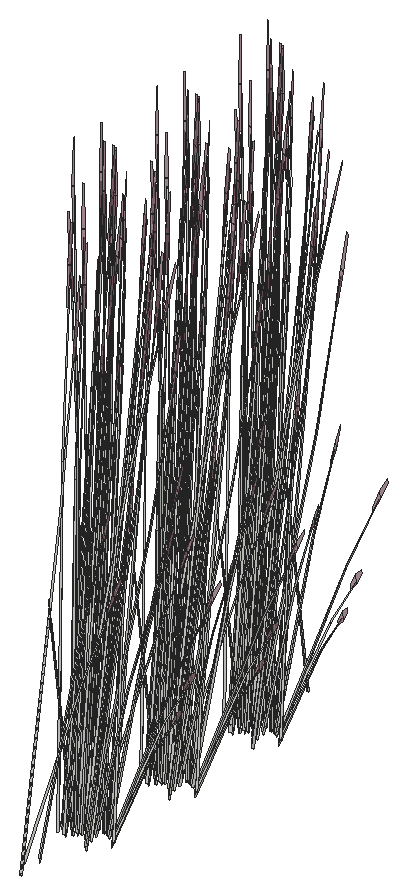
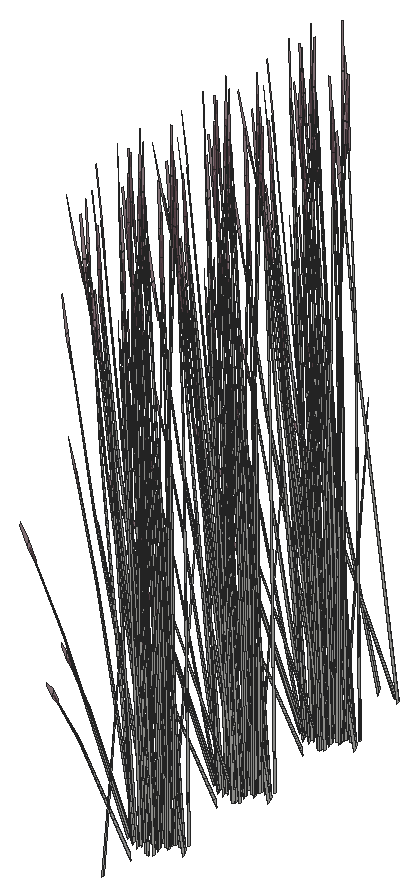
# SketchUp Ruby script. Lengths in inches.
U = 1.inch
M = Sketchup.active_model
def pt(a) = Geom::Point3d.new(a.map { |v| v * U })
def face(e, loops, mat)
  f = e.add_face(loops[0].map { |a| pt(a) })
  loops[1..].each { |l| e.add_face(l.map { |a| pt(a) }).erase! }
  f.material = f.back_material = mat if mat
  f
end
# faces: each face lists its corners as indices into pts; further lists are holes
def faces(e, pts, list, mat = nil) = list.each { |f| face(e, (f[0].is_a?(Array) ? f : [f]).map { |l| l.map { |i| pts[i] } }, mat) }
# xy, xz, yz: faces in a plane at the given z, y or x. An outline is a flat list of corners, or four numbers for a rectangle; further outlines are holes
def ring(l) = l.size == 4 ? [[l[0], l[1]], [l[2], l[1]], [l[2], l[3]], [l[0], l[3]]] : l.each_slice(2).to_a
def flat(e, list, mat, &to3) = list.each { |f| face(e, (f[0].is_a?(Array) ? f : [f]).map { |l| ring(l).map { |u, v| to3.(u, v) } }, mat) }
def xy(e, z, list, mat = nil) = flat(e, list, mat) { |x, y| [x, y, z] }
def xz(e, y, list, mat = nil) = flat(e, list, mat) { |x, z| [x, y, z] }
def yz(e, x, list, mat = nil) = flat(e, list, mat) { |y, z| [x, y, z] }
def lines(e, pts, list) = list.each { |a, b| e.add_line(pt(pts[a]), pt(pts[b])) }
# prism: a flat outline (further loops are holes) pulled along v
def prism(e, loops, v, mat = nil)
  f = face(e, loops, mat); d = Geom::Vector3d.new(v.map { |x| x * U })
  f.pushpull(f.normal.samedirection?(d) ? d.length : -d.length)
end
def box(e, o, s, mat = nil) = prism(e, [[o, [o[0] + s[0], o[1], o[2]], [o[0] + s[0], o[1] + s[1], o[2]], [o[0], o[1] + s[1], o[2]]]], [0, 0, s[2]], mat)
def at(x, y, z, deg = 0) = Geom::Transformation.translation(pt([x, y, z])) * Geom::Transformation.rotation(ORIGIN, Z_AXIS, deg.degrees)
def axes(o, x, y, z) = Geom::Transformation.new([*x, 0, *y, 0, *z, 0, *pt(o).to_a, 1])
def part(name) = M.definitions.add(name)
# library, detail: a bought-in or finely detailed component or shape, given as its bounding box
def library(name, o, s) = part(name).tap { |d| box(d.entities, o, s) }
def detail(e, o, s) = box(e.add_group.entities, o, s)
def put(e, d, t, mat = nil) = e.add_instance(d, t).tap { |i| i.material = mat if mat }
def group(e, t, mat = nil) = e.add_group.tap { |g| g.transformation = t; g.material = mat if mat }.entities
root = M.entities
M.materials.add("LightPink_Translucent").color = [144, 107, 117]
M.materials["LightPink_Translucent"].alpha = 0.75
c1 = part("blade")
p = [[2.15,0.21,22],[0,0.17,0],[0.09,0.45,0],[2.18,0.31,22],[2.29,0.31,22],[0.38,0.45,0],
  [2.48,0.24,33],[2.49,0.24,33],[2.48,0.22,33]]
faces(c1.entities,p,[[0,1,2,3],[4,5,2,3],[6,3,4,7],[8,0,3,6]])
c2 = part("seeds")
p = [[0.3,-0.1,1.38],[-0.01,-0.03,1.59],[-0.01,-0.03,0.03],[0.14,-0.07,-0.07],[0.29,-0.03,3],[0.15,0.01,3.11]]
faces(c2.entities,p,[[0,1,2,3],[1,0,4,5]],"LightPink_Translucent")
c3 = part("blade with seeds")
put(c3.entities,c1,at(0,0,0))
put(c3.entities,c2,axes([2.4,0.25,30.99],[1.5799,-0.05474,1.17369],[-0.12525,1.92788,0.29478],[-0.07173,-0.02425,1.56792]))
put(root,c3,axes([334.9,443.32,49.85],[0.18514,0.35777,-0.61156],[-0.53331,0.12885,-0.16051],[0.02046,0.12115,1.3499]))
put(root,c3,axes([335.47,444.69,50.36],[-0.32378,-0.01225,0.92831],[0.21383,-0.26028,0.51254],[0.12791,0.09247,0.72818]))
put(root,c3,axes([334.77,449.54,50.29],[-0.14352,0.07909,1.26356],[-0.42983,-0.13843,-0.27174],[0.07968,-0.17216,0.54024]))
put(root,c3,axes([334.42,444.06,50.29],[0.00891,-0.12953,1.26356],[0.4258,-0.14469,-0.27174],[0.13144,0.15503,0.54024]))
put(root,c3,axes([335.77,449.78,49.32],[-0.07557,-0.03078,1.55816],[-0.19412,-0.34391,-0.23804],[0.13095,-0.09333,0.26541]))
put(root,c3,axes([332.92,449.85,50.1],[-0.31568,-0.39156,0],[0.52815,-0.21836,-0.456],[0.12029,-0.04973,1.44655]))
put(root,c3,axes([333.35,449.79,49.78],[0.47255,-0.19538,-0.43871],[0.28245,0.35034,0],[0.10763,-0.0445,1.3917]))
put(root,c3,axes([336.15,450.47,50.29],[-0.18038,-0.01157,1.26356],[-0.18479,-0.31048,-0.27174],[0.22159,-0.08783,0.54024]))
put(root,c3,axes([333.91,450.6,49.82],[0.34009,-0.2937,-0.55095],[0.42248,0.26632,-0.1446],[0.13628,-0.07327,1.21613]))
put(root,c3,axes([333.54,450.9375,50.36],[-0.05884,-0.44587,-0.25709],[0.6128,-0.02696,-0.44182],[0.10791,-0.05939,1.41118]))
put(root,c3,axes([333.46,449.95,49.79],[0.47106,0.09668,-0.27372],[-0.11861,0.34048,0.27372],[0.09497,-0.03926,1.22797]))
put(root,c3,axes([333.62,451.29,50.15],[0.56891,0.18939,0.21263],[-0.2738,0.39352,0.44182],[0,-0.09071,1.41855]))
put(root,c3,axes([333.44,451.02,50.4],[-0.54829,0.02412,0.39531],[-0.04958,-0.40041,-0.19025],[0.09816,-0.04058,1.26923]))
put(root,c3,axes([335.24,449.95,50.1],[0.31568,-0.39156,0],[0.52815,0.21836,-0.456],[0.12029,0.04973,1.44655]))
put(root,c3,axes([336.49,451.5,49.75],[-0.3252,0.04689,1.25103],[-0.05176,-0.37326,0.07161],[0.22777,-0.0565,0.71188]))
put(root,c3,axes([337.08,451.17,50],[-0.31304,-0.24986,-0.05733],[0.34284,-0.22894,-0.25992],[0.09714,-0.01612,0.85731]))
put(root,c3,axes([334.21,451.2,49.95],[0,-0.45213,0],[0.63136,0,0],[0,0,1.58567]))
put(root,c3,axes([334.97,450.16,50.19],[-0.47255,-0.19538,0.43871],[0.28245,-0.35034,0],[0.10763,0.0445,1.3917]))
put(root,c3,axes([333.91,450.92,50.09],[-0.41865,0.35461,0.40429],[-0.49737,-0.31303,0.15865],[0.10093,-0.03539,1.40366]))
put(root,c3,axes([333.18,450.33,50.1875],[-0.14586,0.38834,0.15589],[-0.53375,-0.1099,0.31002],[0.0922,-0.00189,1.41735]))
put(root,c3,axes([332.96,450.65,49.41],[-0.49699,0.15644,1.13921],[-0.15819,-0.44887,0.44265],[0.30518,0.00747,1.29573]))
put(root,c3,axes([334.29,450.77,50.3125],[0.09741,-0.34873,0.12794],[0.4759,0.06053,-0.36534],[0.08661,0.03581,1.11991]))
put(root,c3,axes([336.84,451.26,49.32],[-0.02639,-0.05932,1.55816],[0.18302,-0.34702,-0.23804],[0.18462,-0.00499,0.26541]))
put(root,c3,axes([334.09,450.86,50.4],[-0.30332,-0.32798,0.39531],[0.45944,-0.23096,-0.19025],[0.09816,0.04058,1.26923]))
put(root,c3,axes([334.25,450.88,50.36],[0.50979,-0.25942,-0.25709],[0.339,0.36656,-0.44182],[0.12578,0.03723,1.41118]))
put(root,c3,axes([335.53,450.1875,49.78],[0.47255,0.19538,-0.43871],[-0.28245,0.35034,0],[0.10763,0.0445,1.3917]))
put(root,c3,axes([334.63,451.3,49.95],[0.56491,0,0],[0,0.40454,0],[0,0,1.5764]))
put(root,c3,axes([334.79,450.36,50.1875],[-0.54257,0.10371,0.15589],[-0.13397,-0.38597,0.31002],[0.04839,0.05624,1.41735]))
put(root,c3,axes([335.4,450.34,49.79],[0.11861,0.34048,-0.27372],[-0.47106,0.09668,0.27372],[0.09497,0.03926,1.22797]))
put(root,c3,axes([334.45,451.1,50.1],[-0.63817,-0.08233,0.43472],[0.12987,-0.46497,0.17059],[0.09326,0.0449,1.50931]))
put(root,c3,axes([334.56,452.2,49.93],[0.53009,-0.13258,-0.16963],[0.18627,0.38191,0.00007],[0.05851,-0.01465,1.53656]))
put(root,c3,axes([334.62,451.48,49.96],[0.35245,0.2524,0],[-0.35245,0.2524,0],[0,0,1.49564]))
put(root,c3,axes([335.58,451.37,50.1875],[-0.39671,-0.28463,0.15589],[0.39978,-0.27607,0.31002],[-0.04381,0.05813,1.41735]))
put(root,c3,axes([334.84,450.9375,49.82],[0.52523,0.06406,-0.55095],[-0.11084,0.39517,-0.1446],[0.15674,0.04788,1.21613]))
put(root,c3,axes([334.62,451.18,50.4],[0.24498,-0.3521,0.39531],[0.50902,0.16945,-0.19025],[0,0.08116,1.26923]))
put(root,c3,axes([334.52,451.38,50.03],[0,0.45191,-0.04981],[-0.63136,0,0],[0,0.0142,1.58489]))
put(root,c3,axes([334.57,451.0625,49.95],[0.30332,0.32798,-0.39531],[-0.45944,0.23096,0.19025],[0.09816,0.04058,1.26923]))
put(root,c3,axes([335.9,451.38,50.19],[0,-0.39075,0.43871],[0.56491,0,0],[0,0.089,1.3917]))
put(root,c3,axes([334.83,451.26,50.3125],[0.47043,-0.11396,0.12794],[0.16474,0.32541,-0.36534],[0,0.07162,1.11991]))
put(root,c3,axes([336.58,452.06,50.29],[-0.1216,-0.0961,1.26356],[0.15822,-0.31792,-0.27174],[0.24603,0.04307,0.54024]))
put(root,c3,axes([334.4,452.41,49.95],[0.50902,0.17543,0],[-0.24498,0.36452,0],[0,0,1.54589]))
put(root,c3,axes([334.22,452.26,50.02],[0.21952,0.44891,-0.05313],[-0.62724,0.1573,0],[0.00767,0.01568,1.52132]))
put(root,c3,axes([336.29,451.44,50.1],[0.63136,0,0],[0,0.43672,-0.456],[0,0.09947,1.44655]))
put(root,c3,axes([336.03,451.67,49.94],[-0.63105,-0.00312,-0.04397],[0,-0.43672,0.44129],[-0.01983,0.09942,1.3992]))
put(root,c3,axes([334.67,451.29,50.36],[0.56863,0.18645,-0.25709],[-0.2738,0.39352,-0.44182],[0.01787,0.09662,1.41118]))
put(root,c3,axes([335.9,451.73,49.79],[-0.35245,0.2438,-0.27372],[-0.35245,-0.2438,0.27372],[0,0.07853,1.22797]))
put(root,c3,axes([334.61,451.58,49.95],[-0.24498,0.3521,-0.39531],[-0.50902,-0.16945,0.19025],[0,0.08116,1.26923]))
put(root,c3,axes([336.15,451.74,49.78],[0,0.39075,-0.43871],[-0.56491,0,0],[0,0.089,1.3917]))
put(root,c3,axes([335.51,452.97,49.32],[0.03679,-0.05641,1.55816],[0.46313,-0.16615,-0.23804],[0.14041,0.08599,0.26541]))
put(root,c3,axes([334.9,451.6875,49.85],[0.18514,0.35777,-0.61156],[-0.53331,0.12885,-0.16051],[0.02046,0.12115,1.3499]))
put(root,c3,axes([335.47,453.0625,50.36],[-0.32378,-0.01225,0.92831],[0.21383,-0.26028,0.51254],[0.12791,0.09247,0.72818]))
put(root,c3,axes([334.42,452.43,50.29],[0.00891,-0.12953,1.26356],[0.4258,-0.14469,-0.27174],[0.13144,0.15503,0.54024]))
put(root,c3,axes([334.77,459.05,50.29],[-0.14352,0.07909,1.26356],[-0.42983,-0.13843,-0.27174],[0.07968,-0.17216,0.54024]))
put(root,c3,axes([335.77,459.3,49.32],[-0.07557,-0.03078,1.55816],[-0.19412,-0.34391,-0.23804],[0.13095,-0.09333,0.26541]))
put(root,c3,axes([332.92,459.37,50.1],[-0.31568,-0.39156,0],[0.52815,-0.21836,-0.456],[0.12029,-0.04973,1.44655]))
put(root,c3,axes([333.35,459.31,49.78],[0.47255,-0.19538,-0.43871],[0.28245,0.35034,0],[0.10763,-0.0445,1.3917]))
put(root,c3,axes([336.15,459.98,50.29],[-0.18038,-0.01157,1.26356],[-0.18479,-0.31048,-0.27174],[0.22159,-0.08783,0.54024]))
put(root,c3,axes([333.91,460.11,49.82],[0.34009,-0.2937,-0.55095],[0.42248,0.26632,-0.1446],[0.13628,-0.07327,1.21613]))
put(root,c3,axes([333.54,460.45,50.36],[-0.05884,-0.44587,-0.25709],[0.6128,-0.02696,-0.44182],[0.10791,-0.05939,1.41118]))
put(root,c3,axes([333.46,459.46,49.79],[0.47106,0.09668,-0.27372],[-0.11861,0.34048,0.27372],[0.09497,-0.03926,1.22797]))
put(root,c3,axes([333.62,460.8,50.15],[0.56891,0.18939,0.21263],[-0.2738,0.39352,0.44182],[0,-0.09071,1.41855]))
put(root,c3,axes([333.44,460.54,50.4],[-0.54829,0.02412,0.39531],[-0.04958,-0.40041,-0.19025],[0.09816,-0.04058,1.26923]))
put(root,c3,axes([335.24,459.47,50.1],[0.31568,-0.39156,0],[0.52815,0.21836,-0.456],[0.12029,0.04973,1.44655]))
put(root,c3,axes([336.49,461.02,49.75],[-0.3252,0.04689,1.25103],[-0.05176,-0.37326,0.07161],[0.22777,-0.0565,0.71188]))
put(root,c3,axes([337.08,460.68,50],[-0.31304,-0.24986,-0.05733],[0.34284,-0.22894,-0.25992],[0.09714,-0.01612,0.85731]))
put(root,c3,axes([334.21,460.72,49.95],[0,-0.45213,0],[0.63136,0,0],[0,0,1.58567]))
put(root,c3,axes([334.97,459.67,50.19],[-0.47255,-0.19538,0.43871],[0.28245,-0.35034,0],[0.10763,0.0445,1.3917]))
put(root,c3,axes([333.91,460.43,50.09],[-0.41865,0.35461,0.40429],[-0.49737,-0.31303,0.15865],[0.10093,-0.03539,1.40366]))
put(root,c3,axes([333.18,459.85,50.1875],[-0.14586,0.38834,0.15589],[-0.53375,-0.1099,0.31002],[0.0922,-0.00189,1.41735]))
put(root,c3,axes([332.96,460.16,49.41],[-0.49699,0.15644,1.13921],[-0.15819,-0.44887,0.44265],[0.30518,0.00747,1.29573]))
put(root,c3,axes([334.29,460.28,50.3125],[0.09741,-0.34873,0.12794],[0.4759,0.06053,-0.36534],[0.08661,0.03581,1.11991]))
put(root,c3,axes([336.84,460.77,49.32],[-0.02639,-0.05932,1.55816],[0.18302,-0.34702,-0.23804],[0.18462,-0.00499,0.26541]))
put(root,c3,axes([334.09,460.37,50.4],[-0.30332,-0.32798,0.39531],[0.45944,-0.23096,-0.19025],[0.09816,0.04058,1.26923]))
put(root,c3,axes([334.25,460.39,50.36],[0.50979,-0.25942,-0.25709],[0.339,0.36656,-0.44182],[0.12578,0.03723,1.41118]))
put(root,c3,axes([335.53,459.7,49.78],[0.47255,0.19538,-0.43871],[-0.28245,0.35034,0],[0.10763,0.0445,1.3917]))
put(root,c3,axes([334.63,460.82,49.95],[0.56491,0,0],[0,0.40454,0],[0,0,1.5764]))
put(root,c3,axes([334.79,459.87,50.1875],[-0.54257,0.10371,0.15589],[-0.13397,-0.38597,0.31002],[0.04839,0.05624,1.41735]))
put(root,c3,axes([335.4,459.85,49.79],[0.11861,0.34048,-0.27372],[-0.47106,0.09668,0.27372],[0.09497,0.03926,1.22797]))
put(root,c3,axes([334.45,460.61,50.1],[-0.63817,-0.08233,0.43472],[0.12987,-0.46497,0.17059],[0.09326,0.0449,1.50931]))
put(root,c3,axes([334.56,461.71,49.93],[0.53009,-0.13258,-0.16963],[0.18627,0.38191,0.00007],[0.05851,-0.01465,1.53656]))
put(root,c3,axes([334.62,460.99,49.96],[0.35245,0.2524,0],[-0.35245,0.2524,0],[0,0,1.49564]))
put(root,c3,axes([335.58,460.88,50.1875],[-0.39671,-0.28463,0.15589],[0.39978,-0.27607,0.31002],[-0.04381,0.05813,1.41735]))
put(root,c3,axes([334.84,460.45,49.82],[0.52523,0.06406,-0.55095],[-0.11084,0.39517,-0.1446],[0.15674,0.04788,1.21613]))
put(root,c3,axes([334.62,460.7,50.4],[0.24498,-0.3521,0.39531],[0.50902,0.16945,-0.19025],[0,0.08116,1.26923]))
put(root,c3,axes([334.52,460.9,50.03],[0,0.45191,-0.04981],[-0.63136,0,0],[0,0.0142,1.58489]))
put(root,c3,axes([334.57,460.58,49.95],[0.30332,0.32798,-0.39531],[-0.45944,0.23096,0.19025],[0.09816,0.04058,1.26923]))
put(root,c3,axes([335.9,460.89,50.19],[0,-0.39075,0.43871],[0.56491,0,0],[0,0.089,1.3917]))
put(root,c3,axes([334.83,460.78,50.3125],[0.47043,-0.11396,0.12794],[0.16474,0.32541,-0.36534],[0,0.07162,1.11991]))
put(root,c3,axes([336.58,461.57,50.29],[-0.1216,-0.0961,1.26356],[0.15822,-0.31792,-0.27174],[0.24603,0.04307,0.54024]))
put(root,c3,axes([334.4,461.92,49.95],[0.50902,0.17543,0],[-0.24498,0.36452,0],[0,0,1.54589]))
put(root,c3,axes([334.22,461.77,50.02],[0.21952,0.44891,-0.05313],[-0.62724,0.1573,0],[0.00767,0.01568,1.52132]))
put(root,c3,axes([336.29,460.96,50.1],[0.63136,0,0],[0,0.43672,-0.456],[0,0.09947,1.44655]))
put(root,c3,axes([336.03,461.18,49.94],[-0.63105,-0.00312,-0.04397],[0,-0.43672,0.44129],[-0.01983,0.09942,1.3992]))
put(root,c3,axes([334.67,460.8,50.36],[0.56863,0.18645,-0.25709],[-0.2738,0.39352,-0.44182],[0.01787,0.09662,1.41118]))
put(root,c3,axes([335.9,461.25,49.79],[-0.35245,0.2438,-0.27372],[-0.35245,-0.2438,0.27372],[0,0.07853,1.22797]))
put(root,c3,axes([334.61,461.1,49.95],[-0.24498,0.3521,-0.39531],[-0.50902,-0.16945,0.19025],[0,0.08116,1.26923]))
put(root,c3,axes([336.15,461.26,49.78],[0,0.39075,-0.43871],[-0.56491,0,0],[0,0.089,1.3917]))
put(root,c3,axes([335.51,462.48,49.32],[0.03679,-0.05641,1.55816],[0.46313,-0.16615,-0.23804],[0.14041,0.08599,0.26541]))
put(root,c3,axes([334.9,461.2,49.85],[0.18514,0.35777,-0.61156],[-0.53331,0.12885,-0.16051],[0.02046,0.12115,1.3499]))
put(root,c3,axes([335.47,462.58,50.36],[-0.32378,-0.01225,0.92831],[0.21383,-0.26028,0.51254],[0.12791,0.09247,0.72818]))
put(root,c3,axes([334.42,461.95,50.29],[0.00891,-0.12953,1.26356],[0.4258,-0.14469,-0.27174],[0.13144,0.15503,0.54024]))
put(root,c3,axes([334.77,468.61,50.29],[-0.14352,0.07909,1.26356],[-0.42983,-0.13843,-0.27174],[0.07968,-0.17216,0.54024]))
put(root,c3,axes([335.77,468.85,49.32],[-0.07557,-0.03078,1.55816],[-0.19412,-0.34391,-0.23804],[0.13095,-0.09333,0.26541]))
put(root,c3,axes([332.92,468.93,50.1],[-0.31568,-0.39156,0],[0.52815,-0.21836,-0.456],[0.12029,-0.04973,1.44655]))
put(root,c3,axes([333.35,468.86,49.78],[0.47255,-0.19538,-0.43871],[0.28245,0.35034,0],[0.10763,-0.0445,1.3917]))
put(root,c3,axes([336.15,469.54,50.29],[-0.18038,-0.01157,1.26356],[-0.18479,-0.31048,-0.27174],[0.22159,-0.08783,0.54024]))
put(root,c3,axes([333.91,469.67,49.82],[0.34009,-0.2937,-0.55095],[0.42248,0.26632,-0.1446],[0.13628,-0.07327,1.21613]))
put(root,c3,axes([333.54,470.01,50.36],[-0.05884,-0.44587,-0.25709],[0.6128,-0.02696,-0.44182],[0.10791,-0.05939,1.41118]))
put(root,c3,axes([333.46,469.02,49.79],[0.47106,0.09668,-0.27372],[-0.11861,0.34048,0.27372],[0.09497,-0.03926,1.22797]))
put(root,c3,axes([333.62,470.36,50.15],[0.56891,0.18939,0.21263],[-0.2738,0.39352,0.44182],[0,-0.09071,1.41855]))
put(root,c3,axes([333.44,470.09,50.4],[-0.54829,0.02412,0.39531],[-0.04958,-0.40041,-0.19025],[0.09816,-0.04058,1.26923]))
put(root,c3,axes([335.24,469.02,50.1],[0.31568,-0.39156,0],[0.52815,0.21836,-0.456],[0.12029,0.04973,1.44655]))
put(root,c3,axes([336.49,470.57,49.75],[-0.3252,0.04689,1.25103],[-0.05176,-0.37326,0.07161],[0.22777,-0.0565,0.71188]))
put(root,c3,axes([337.08,470.24,50],[-0.31304,-0.24986,-0.05733],[0.34284,-0.22894,-0.25992],[0.09714,-0.01612,0.85731]))
put(root,c3,axes([334.21,470.27,49.95],[0,-0.45213,0],[0.63136,0,0],[0,0,1.58567]))
put(root,c3,axes([334.97,469.23,50.19],[-0.47255,-0.19538,0.43871],[0.28245,-0.35034,0],[0.10763,0.0445,1.3917]))
put(root,c3,axes([333.91,469.99,50.09],[-0.41865,0.35461,0.40429],[-0.49737,-0.31303,0.15865],[0.10093,-0.03539,1.40366]))
put(root,c3,axes([333.18,469.4,50.1875],[-0.14586,0.38834,0.15589],[-0.53375,-0.1099,0.31002],[0.0922,-0.00189,1.41735]))
put(root,c3,axes([332.96,469.72,49.41],[-0.49699,0.15644,1.13921],[-0.15819,-0.44887,0.44265],[0.30518,0.00747,1.29573]))
put(root,c3,axes([334.29,469.84,50.3125],[0.09741,-0.34873,0.12794],[0.4759,0.06053,-0.36534],[0.08661,0.03581,1.11991]))
put(root,c3,axes([336.84,470.33,49.32],[-0.02639,-0.05932,1.55816],[0.18302,-0.34702,-0.23804],[0.18462,-0.00499,0.26541]))
put(root,c3,axes([334.09,469.93,50.4],[-0.30332,-0.32798,0.39531],[0.45944,-0.23096,-0.19025],[0.09816,0.04058,1.26923]))
put(root,c3,axes([334.25,469.95,50.36],[0.50979,-0.25942,-0.25709],[0.339,0.36656,-0.44182],[0.12578,0.03723,1.41118]))
put(root,c3,axes([335.53,469.26,49.78],[0.47255,0.19538,-0.43871],[-0.28245,0.35034,0],[0.10763,0.0445,1.3917]))
put(root,c3,axes([334.63,470.375,49.95],[0.56491,0,0],[0,0.40454,0],[0,0,1.5764]))
put(root,c3,axes([334.79,469.43,50.1875],[-0.54257,0.10371,0.15589],[-0.13397,-0.38597,0.31002],[0.04839,0.05624,1.41735]))
put(root,c3,axes([335.4,469.41,49.79],[0.11861,0.34048,-0.27372],[-0.47106,0.09668,0.27372],[0.09497,0.03926,1.22797]))
put(root,c3,axes([334.45,470.17,50.1],[-0.63817,-0.08233,0.43472],[0.12987,-0.46497,0.17059],[0.09326,0.0449,1.50931]))
put(root,c3,axes([334.56,471.27,49.93],[0.53009,-0.13258,-0.16963],[0.18627,0.38191,0.00007],[0.05851,-0.01465,1.53656]))
put(root,c3,axes([334.62,470.55,49.96],[0.35245,0.2524,0],[-0.35245,0.2524,0],[0,0,1.49564]))
put(root,c3,axes([335.58,470.4375,50.1875],[-0.39671,-0.28463,0.15589],[0.39978,-0.27607,0.31002],[-0.04381,0.05813,1.41735]))
put(root,c3,axes([334.84,470.01,49.82],[0.52523,0.06406,-0.55095],[-0.11084,0.39517,-0.1446],[0.15674,0.04788,1.21613]))
put(root,c3,axes([334.62,470.25,50.4],[0.24498,-0.3521,0.39531],[0.50902,0.16945,-0.19025],[0,0.08116,1.26923]))
put(root,c3,axes([334.52,470.45,50.03],[0,0.45191,-0.04981],[-0.63136,0,0],[0,0.0142,1.58489]))
put(root,c3,axes([334.57,470.13,49.95],[0.30332,0.32798,-0.39531],[-0.45944,0.23096,0.19025],[0.09816,0.04058,1.26923]))
put(root,c3,axes([335.9,470.45,50.19],[0,-0.39075,0.43871],[0.56491,0,0],[0,0.089,1.3917]))
put(root,c3,axes([334.83,470.33,50.3125],[0.47043,-0.11396,0.12794],[0.16474,0.32541,-0.36534],[0,0.07162,1.11991]))
put(root,c3,axes([336.58,471.125,50.29],[-0.1216,-0.0961,1.26356],[0.15822,-0.31792,-0.27174],[0.24603,0.04307,0.54024]))
put(root,c3,axes([334.4,471.48,49.95],[0.50902,0.17543,0],[-0.24498,0.36452,0],[0,0,1.54589]))
put(root,c3,axes([334.22,471.33,50.02],[0.21952,0.44891,-0.05313],[-0.62724,0.1573,0],[0.00767,0.01568,1.52132]))
put(root,c3,axes([336.29,470.52,50.1],[0.63136,0,0],[0,0.43672,-0.456],[0,0.09947,1.44655]))
put(root,c3,axes([336.03,470.74,49.94],[-0.63105,-0.00312,-0.04397],[0,-0.43672,0.44129],[-0.01983,0.09942,1.3992]))
put(root,c3,axes([334.67,470.36,50.36],[0.56863,0.18645,-0.25709],[-0.2738,0.39352,-0.44182],[0.01787,0.09662,1.41118]))
put(root,c3,axes([335.9,470.8,49.79],[-0.35245,0.2438,-0.27372],[-0.35245,-0.2438,0.27372],[0,0.07853,1.22797]))
put(root,c3,axes([334.61,470.65,49.95],[-0.24498,0.3521,-0.39531],[-0.50902,-0.16945,0.19025],[0,0.08116,1.26923]))
put(root,c3,axes([336.15,470.8125,49.78],[0,0.39075,-0.43871],[-0.56491,0,0],[0,0.089,1.3917]))
put(root,c3,axes([334.77,476.41,50.29],[-0.14352,0.07909,1.26356],[-0.42983,-0.13843,-0.27174],[0.07968,-0.17216,0.54024]))
put(root,c3,axes([335.51,472.04,49.32],[0.03679,-0.05641,1.55816],[0.46313,-0.16615,-0.23804],[0.14041,0.08599,0.26541]))
